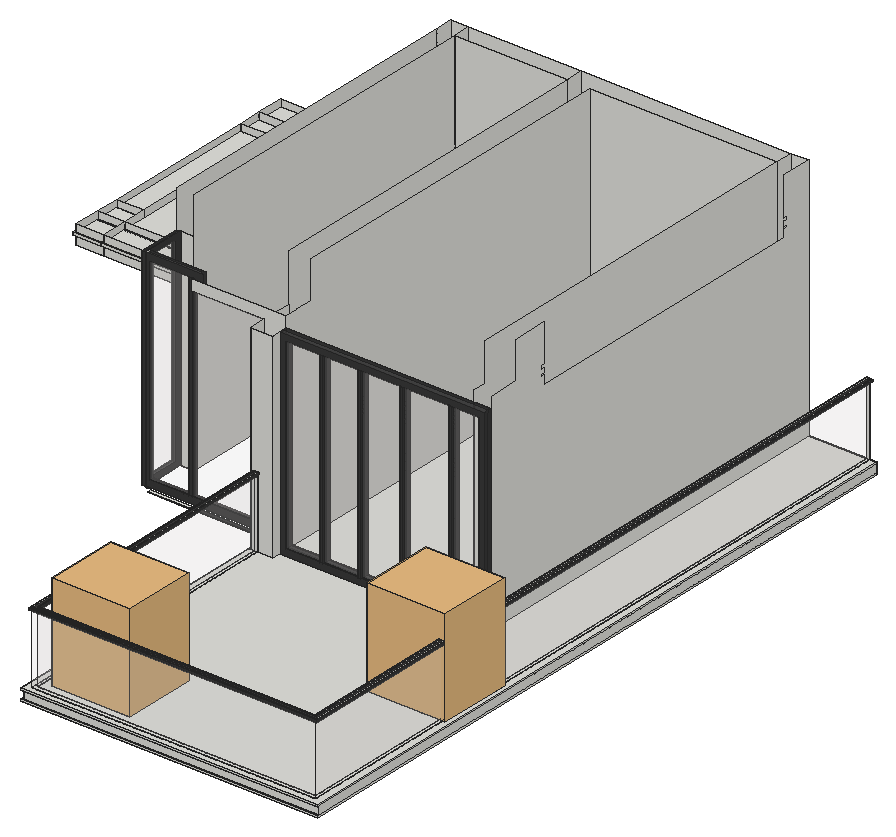
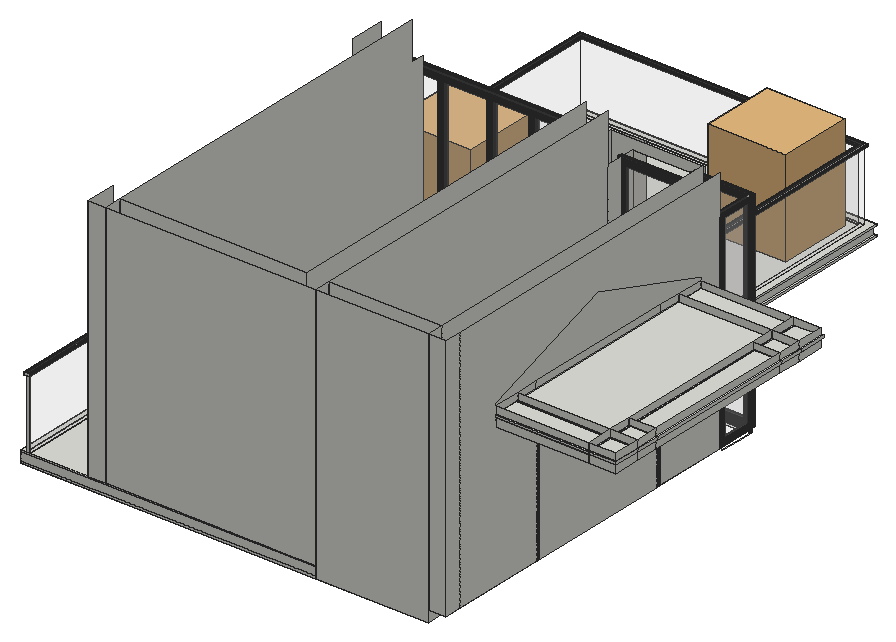
# SketchUp Ruby script. Lengths in inches.
U = 1.inch
M = Sketchup.active_model
def pt(a) = Geom::Point3d.new(a.map { |v| v * U })
def face(e, loops, mat)
  f = e.add_face(loops[0].map { |a| pt(a) })
  loops[1..].each { |l| e.add_face(l.map { |a| pt(a) }).erase! }
  f.material = f.back_material = mat if mat
  f
end
# faces: each face lists its corners as indices into pts; further lists are holes
def faces(e, pts, list, mat = nil) = list.each { |f| face(e, (f[0].is_a?(Array) ? f : [f]).map { |l| l.map { |i| pts[i] } }, mat) }
# xy, xz, yz: faces in a plane at the given z, y or x. An outline is a flat list of corners, or four numbers for a rectangle; further outlines are holes
def ring(l) = l.size == 4 ? [[l[0], l[1]], [l[2], l[1]], [l[2], l[3]], [l[0], l[3]]] : l.each_slice(2).to_a
def flat(e, list, mat, &to3) = list.each { |f| face(e, (f[0].is_a?(Array) ? f : [f]).map { |l| ring(l).map { |u, v| to3.(u, v) } }, mat) }
def xy(e, z, list, mat = nil) = flat(e, list, mat) { |x, y| [x, y, z] }
def xz(e, y, list, mat = nil) = flat(e, list, mat) { |x, z| [x, y, z] }
def yz(e, x, list, mat = nil) = flat(e, list, mat) { |y, z| [x, y, z] }
def lines(e, pts, list) = list.each { |a, b| e.add_line(pt(pts[a]), pt(pts[b])) }
# prism: a flat outline (further loops are holes) pulled along v
def prism(e, loops, v, mat = nil)
  f = face(e, loops, mat); d = Geom::Vector3d.new(v.map { |x| x * U })
  f.pushpull(f.normal.samedirection?(d) ? d.length : -d.length)
end
def box(e, o, s, mat = nil) = prism(e, [[o, [o[0] + s[0], o[1], o[2]], [o[0] + s[0], o[1] + s[1], o[2]], [o[0], o[1] + s[1], o[2]]]], [0, 0, s[2]], mat)
def at(x, y, z, deg = 0) = Geom::Transformation.translation(pt([x, y, z])) * Geom::Transformation.rotation(ORIGIN, Z_AXIS, deg.degrees)
def axes(o, x, y, z) = Geom::Transformation.new([*x, 0, *y, 0, *z, 0, *pt(o).to_a, 1])
def part(name) = M.definitions.add(name)
# library, detail: a bought-in or finely detailed component or shape, given as its bounding box
def library(name, o, s) = part(name).tap { |d| box(d.entities, o, s) }
def detail(e, o, s) = box(e.add_group.entities, o, s)
def put(e, d, t, mat = nil) = e.add_instance(d, t).tap { |i| i.material = mat if mat }
def group(e, t, mat = nil) = e.add_group.tap { |g| g.transformation = t; g.material = mat if mat }.entities
root = M.entities
M.materials.add("Glass Thin Clear 001").color = [255, 250, 250]
M.materials["Glass Thin Clear 001"].alpha = 0.1
M.materials.add("[Color M07]").color = [58, 58, 58]
c1 = library("False Aralia 002",[-20.33,-19.19,0],[40.48,38.23,49.87])
xy(root,243.5,[[208.4375,269.93,210.8125,270.37],[208.4375,270.37,210.8125,272.05]],"[Color M07]")
xy(root,246,[[208.375,108.3125,209.4375,255.6875],[209.4375,108.3125,353,109.375],[353,108.3125,362,109.375],[209.4375,109.375,353,255.6875],[353,109.375,362,469.5625],
  [208.375,255.6875,209.4375,264.6875],[209.4375,255.6875,220.8125,264.6875],[220.8125,255.6875,353,264.6875],[208.375,264.6875,209.4375,271.43],[[209.4375,264.6875,209.4375,460.5625,211.8125,460.5625,211.8125,469.5625,220.8125,469.5625,220.8125,264.6875],[210.9375,269.93,213.3125,272.05]],
  [220.8125,264.6875,353,460.5625],[208.375,271.43,209.4375,280.43],[151,460.5625,209.4375,469.5625],[209.4375,460.5625,211.8125,469.5625],[220.8125,460.5625,353,469.5625]])
xy(root,246,[[210.9375,269.93,213.3125,271.43],[210.9375,271.43,213.3125,272.05]],"[Color M07]")
xy(root,246.9375,[[208.375,108.3125,209.4375,271.43],[209.4375,108.3125,362,109.375],[209.4375,109.375,362,469.5625],[208.375,271.43,209.4375,280.43]])
xy(root,249.5,[[166.4375,269.93,168.4375,272.05],[144.9375,270.37,166.4375,272.05]])
xy(root,249.5,[[144.9375,269.93,166.4375,270.37],[168.4375,269.93,208.4375,270.37],[168.4375,270.37,208.4375,272.05]],"[Color M07]")
xy(root,250.36,[[142,272.01,142.4375,272.05],[142.4375,272.01,144.125,272.05],[142,272.05,142.4375,280.43],[142,280.43,142.4375,290.47]])
xy(root,251.125,[[208.375,108.3125,209.4375,271.43],[209.4375,108.3125,362,109.375],[209.4375,109.375,362,469.5625],[208.375,271.43,209.4375,280.43]])
xy(root,252,[[208.375,108.3125,362,108.3125,362,469.5625,358.82,469.5625,358.82,111.49,211.55,111.49,211.55,255.6875,208.375,255.6875],[211.55,111.49,211.55,255.6875,213.29,255.6875,213.29,113.23,357.09,113.23,357.09,469.5625,358.82,469.5625,358.82,111.49],[213.29,113.23,357.09,113.23,357.09,469.5625,326.84,469.5625,326.84,264.6875,220.8125,264.6875,220.8125,264.4375,326.84,264.4375,326.84,260.1875,220.8125,260.1875,220.8125,255.6875,213.29,255.6875],[208.375,255.6875,209.4375,264.6875],[209.4375,255.6875,220.8125,264.6875],
  [208.375,264.6875,209.4375,269.93],[209.4375,264.6875,209.4375,269.93,210.9375,269.93,210.9375,272.05,209.4375,272.05,209.4375,469.5625,317.84,469.5625,317.84,460.5625,220.8125,460.5625,220.8125,264.6875],[220.8125,264.6875,317.84,460.5625],[317.84,264.6875,326.84,469.5625],[209.4375,269.93,210.9375,271.43],
  [209.4375,271.43,210.9375,272.05],[208.375,272.05,209.4375,280.43],[142,292.12,151,469.5625]])
xy(root,252,[[220.8125,260.1875,317.84,262.625],[317.84,260.1875,326.84,262.625],[220.8125,262.625,317.84,264.4375],[317.84,262.625,326.84,264.4375],[142,269.93,143.5,271.43],
  [143.5,269.93,144.125,271.43],[144.125,269.93,208.375,271.43],[208.375,269.93,209.4375,271.43],[142,271.43,143.5,272.05],[143.5,271.43,144.125,272.05],
  [144.125,271.43,208.375,272.05],[208.375,271.43,209.4375,272.05],[142,272.05,143.5,280.43],[143.5,272.05,144.125,280.43],[142,280.43,143.5,292.12],
  [143.5,280.43,144.125,292.12]],"[Color M07]")
xy(root,254.83,[[142,273.2,142.4375,280.43],[142.4375,273.2,144.125,280.43],[142,280.43,142.4375,289.29],[142.4375,280.43,144.125,289.29]],"[Color M07]")
xy(root,255.11,[[241.62,260.1875,243.38,264.4375],[261.3,260.1875,263.07,264.4375],[283.05,260.1875,284.82,264.4375],[308.3125,260.1875,310.08,264.4375]])
xy(root,255.11,[[223.93,260.1875,241.62,261.1875],[243.38,260.1875,261.3,261.1875],[263.07,260.1875,283.05,261.1875],[284.82,260.1875,308.3125,261.1875],[310.08,260.1875,317.84,261.1875],
  [317.84,260.1875,323.73,261.1875],[223.93,261.1875,241.62,264.4375],[243.38,261.1875,261.3,264.4375],[263.07,261.1875,283.05,264.4375],[284.82,261.1875,308.3125,264.4375],
  [310.08,261.1875,317.84,264.4375],[317.84,261.1875,323.73,264.4375]],"[Color M07]")
xy(root,255.5,[[166.4375,269.93,168.4375,272.05]])
xy(root,255.5,[[145.94,269.93,166.4375,270.37],[168.4375,269.93,207.43,270.37],[145.94,270.37,166.4375,272.05],[168.4375,270.37,207.43,272.05]],"[Color M07]")
xy(root,288,[[211.55,111.49,211.55,255.6875,213.29,255.6875,213.29,113.23,357.09,113.23,357.09,469.5625,358.82,469.5625,358.82,111.49]])
xy(root,288,[[[210.93,110.87,210.93,256.3125,213.91,256.3125,213.91,113.85,356.46,113.85,356.46,470.1875,359.44,470.1875,359.44,110.87],[211.55,111.49,358.82,111.49,358.82,469.5625,357.09,469.5625,357.09,113.23,213.29,113.23,213.29,255.6875,211.55,255.6875]]],"[Color M07]")
xy(root,289.1875,[[[210.93,110.87,359.44,110.87,359.44,470.1875,356.46,470.1875,356.46,113.85,213.91,113.85,213.91,256.3125,210.93,256.3125],[211.55,111.49,211.55,255.6875,213.29,255.6875,213.29,113.23,357.09,113.23,357.09,469.5625,358.82,469.5625,358.82,111.49]],[211.55,111.49,358.82,111.49,358.82,469.5625,357.09,469.5625,357.09,113.23,213.29,113.23,213.29,255.6875,211.55,255.6875]],"[Color M07]")
xy(root,321.57,[[110.9,331.125,112.77,331.5625],[110.9,331.5625,112.77,332.75],[110.9,409.3125,112.77,409.75],[110.9,409.75,112.77,410.9375]])
xy(root,321.57,[[99.31,331.125,110.9,331.5625],[112.77,331.125,137.69,331.5625],[99.31,331.5625,110.9,332.75],[112.77,331.5625,137.69,332.75],[99.31,409.3125,110.9,409.75],
  [112.77,409.3125,137.69,409.75],[99.31,409.75,110.9,410.9375],[112.77,409.75,137.69,410.9375]],"[Color M07]")
xy(root,325.875,[[79.875,305,94,319.125],[94,305,142,319.125],[79.875,319.125,79.875,331.125,86,331.125,86,330.5625,94,330.5625,94,319.125],[94,319.125,94,330.5625,95,330.5625,95,331.125,142,331.125,142,319.125],[86,330.5625,94,331.125],
  [94,330.5625,95,331.125],[79.875,331.125,79.875,411.25,94,411.25,94,411.125,86,411.125,86,331.125],[86,331.125,94,411.125],[94,331.125,95,411.125],[95,332.75,142,333.43],
  [95,333.43,142,409.3125],[95,410.9375,95,411.125,94,411.125,94,411.25,142,411.25,142,410.9375],[79.875,411.25,94,423.25],[94,411.25,142,423.25],[79.875,423.25,94,437.375],
  [94,423.25,142,437.375]])
xy(root,325.875,[[95,331.125,142,332.125],[95,332.125,142,332.75],[95,409.3125,142,410.3125],[95,410.3125,142,410.9375]],"[Color M07]")
xy(root,330.53,[[79.0625,304.1875,79.0625,318.3125,79.875,318.3125,79.875,305,93.1875,305,93.1875,304.1875],[93.1875,304.1875,142,305],[79.875,305,93.1875,318.3125],[93.1875,305,94,318.3125],[94,305,142,318.3125],
  [79.0625,318.3125,79.875,319.125],[79.875,318.3125,93.1875,319.125],[93.1875,318.3125,94,319.125],[94,318.3125,142,319.125],[79.0625,319.125,79.875,331.125],
  [79.875,319.125,93.1875,331.125],[93.1875,319.125,94,331.125],[94,319.125,142,423.25],[79.0625,331.125,79.875,411.25],[79.875,331.125,93.1875,411.25],
  [93.1875,331.125,94,411.25],[79.0625,411.25,79.875,424.0625],[79.875,411.25,93.1875,423.25],[93.1875,411.25,94,423.25],[79.875,423.25,93.1875,424.0625],
  [93.1875,423.25,94,424.0625],[94,423.25,142,424.0625],[79.0625,424.0625,79.0625,438.1875,93.1875,438.1875,93.1875,437.375,79.875,437.375,79.875,424.0625],[79.875,424.0625,93.1875,437.375],[93.1875,424.0625,94,437.375],
  [94,424.0625,142,437.375],[93.1875,437.375,94,438.1875],[94,437.375,142,438.1875]])
xy(root,331.84,[[79.0625,304.1875,93.1875,304.1875,93.1875,305,79.875,305,79.875,318.3125,79.0625,318.3125],[93.1875,304.1875,142,305],[79.875,305,93.1875,318.3125],[93.1875,305,94,318.3125],[94,305,142,318.3125],
  [79.0625,318.3125,79.875,319.125],[79.875,318.3125,93.1875,319.125],[93.1875,318.3125,94,319.125],[94,318.3125,142,319.125],[79.0625,319.125,79.875,331.125],
  [79.875,319.125,93.1875,331.125],[93.1875,319.125,94,331.125],[94,319.125,142,423.25],[79.0625,331.125,79.875,411.25],[79.875,331.125,93.1875,411.25],
  [93.1875,331.125,94,411.25],[79.0625,411.25,79.875,424.0625],[79.875,411.25,93.1875,423.25],[93.1875,411.25,94,423.25],[79.875,423.25,93.1875,424.0625],
  [93.1875,423.25,94,424.0625],[94,423.25,142,424.0625],[79.0625,424.0625,79.875,424.0625,79.875,437.375,93.1875,437.375,93.1875,438.1875,79.0625,438.1875],[79.875,424.0625,93.1875,437.375],[93.1875,424.0625,94,437.375],
  [94,424.0625,142,437.375],[93.1875,437.375,94,438.1875],[94,437.375,142,438.1875]])
xz(root,108.3125,[[208.375,246,362,246.9375],[208.375,251.125,362,252]])
xz(root,109.375,[[209.4375,246.9375,362,251.125]])
xz(root,110.87,[[210.93,288,359.44,289.1875]],"[Color M07]")
xz(root,111.49,[[211.55,288,358.82,289.1875]])
xz(root,111.49,[[211.55,252,358.82,288]],"Glass Thin Clear 001")
xz(root,113.23,[[213.29,288,357.09,289.1875]])
xz(root,113.23,[[213.29,252,357.09,288]],"Glass Thin Clear 001")
xz(root,113.85,[[213.91,288,356.46,289.1875]],"[Color M07]")
xz(root,255.6875,[[209.4375,252,211.55,252,211.55,289.1875,213.29,289.1875,213.29,252,220.8125,252,220.8125,354.57,209.4375,354.57],[211.55,252,213.29,288],[211.55,288,213.29,289.1875]])
xz(root,256.3125,[[210.93,288,213.91,289.1875]])
xz(root,260.1875,[[[220.8125,252,326.84,354.57],[223.93,255.11,323.73,351.46]],[241.62,255.11,243.38,351.46],[261.3,255.11,263.07,351.46],[283.05,255.11,284.82,351.46],[308.3125,255.11,310.08,351.46]],"[Color M07]")
xz(root,261.1875,[[223.93,255.11,241.62,351.46],[243.38,255.11,261.3,351.46],[263.07,255.11,283.05,351.46],[284.82,255.11,308.3125,351.46],[310.08,255.11,323.73,351.46]],"Glass Thin Clear 001")
xz(root,262.625,[[220.8125,252,326.84,354.57]],"Glass Thin Clear 001")
xz(root,264.4375,[[[220.8125,252,326.84,354.57],[223.93,255.11,323.73,351.46]],[241.62,255.11,243.38,351.46],[261.3,255.11,263.07,351.46],[283.05,255.11,284.82,351.46],[308.3125,255.11,310.08,351.46]],"[Color M07]")
xz(root,264.6875,[[209.4375,252,209.4375,354.57,171.8125,354.57,171.8125,360,220.8125,360,220.8125,252],[317.84,252,326.84,354.57]])
xz(root,269.93,[[142,252,144.125,360.375],[[144.125,252,210.9375,252,210.9375,354.57,173.3125,354.57,173.3125,360,173.125,360,173.125,360.375,144.125,360.375],[145.94,255.5,145.94,356.87,169.62,356.87,169.62,356.5,169.81,356.5,169.81,351.07,207.43,351.07,207.43,255.5]],[166.4375,255.5,168.4375,356.87]],"[Color M07]")
xz(root,270.37,[[145.94,255.5,166.4375,356.87],[168.4375,255.5,207.43,255.5,207.43,351.07,169.81,351.07,169.81,356.5,169.62,356.5,169.62,356.87,168.4375,356.87]],"Glass Thin Clear 001")
xz(root,271.43,[[208.375,246,209.4375,246.9375],[208.375,251.125,209.4375,252]])
xz(root,271.43,[[143.5,252,143.5,360.375,171.625,360.375,171.625,360,171.8125,360,171.8125,354.57,210.9375,354.57,210.9375,252]],"Glass Thin Clear 001")
xz(root,272.05,[[142,250.36,144.125,252],[[144.125,252,144.125,360.375,173.125,360.375,173.125,360,173.3125,360,173.3125,354.57,210.9375,354.57,210.9375,252],[145.94,255.5,207.43,255.5,207.43,351.07,169.81,351.07,169.81,356.5,169.62,356.5,169.62,356.87,145.94,356.87]],[166.4375,255.5,168.4375,356.87]],"[Color M07]")
xz(root,273.2,[[142,254.83,142.4375,357.54],[142.4375,254.83,144.125,357.54]],"[Color M07]")
xz(root,280.43,[[208.375,246,209.4375,246.9375],[208.375,251.125,209.4375,252]])
xz(root,289.29,[[142,254.83,142.4375,357.54],[142.4375,254.83,144.125,357.54]],"[Color M07]")
xz(root,292.12,[[144.125,252,151,360.375]])
xz(root,292.12,[[142,252,143.5,360.375],[143.5,252,144.125,360.375]],"[Color M07]")
xz(root,304.1875,[[79.0625,330.53,93.1875,331.84],[93.1875,330.53,142,331.84]])
xz(root,305,[[79.875,325.875,94,330.53],[94,325.875,142,330.53],[79.875,331.84,94,335.4],[94,331.84,142,335.4]])
xz(root,318.3125,[[79.0625,330.53,93.1875,331.84],[93.1875,330.53,142,331.84]])
xz(root,319.125,[[79.875,325.875,94,330.53],[94,325.875,142,330.53],[79.875,331.84,94,335.4],[94,331.84,142,335.4]])
xz(root,331.125,[[79.875,325.875,94,330.53],[79.0625,330.53,93.1875,331.84],[79.875,331.84,94,335.4]])
xz(root,411.25,[[79.875,325.875,94,330.53],[79.0625,330.53,93.1875,331.84],[79.875,331.84,94,335.4]])
xz(root,423.25,[[79.875,325.875,94,330.53],[94,325.875,142,330.53],[79.875,331.84,94,335.4],[94,331.84,142,335.4]])
xz(root,424.0625,[[79.0625,330.53,93.1875,331.84],[93.1875,330.53,142,331.84]])
xz(root,437.375,[[79.875,325.875,94,330.53],[94,325.875,142,330.53],[79.875,331.84,94,335.4],[94,331.84,142,335.4]])
xz(root,438.1875,[[79.0625,330.53,93.1875,331.84],[93.1875,330.53,142,331.84]])
xz(root,460.5625,[[151,246,209.4375,379.5625],[220.8125,252,317.84,379.5625]])
xz(root,469.5625,[[151,246,209.4375,379.5625],[209.4375,246,362,246.9375],[209.4375,246.9375,362,251.125],[209.4375,251.125,362,252],[142,252,151,379.5625],
  [209.4375,252,317.84,379.5625],[317.84,252,326.84,379.5625],[357.09,252,358.82,288],[357.09,288,358.82,289.1875]])
xz(root,470.1875,[[356.46,288,359.44,289.1875]])
yz(root,79.0625,[[304.1875,330.53,318.3125,331.84],[318.3125,330.53,331.125,331.84],[331.125,330.53,411.25,331.84],[411.25,330.53,424.0625,331.84],[424.0625,330.53,438.1875,331.84]])
yz(root,79.875,[[305,325.875,319.125,330.53],[319.125,325.875,331.125,330.53],[331.125,325.875,411.25,330.53],[411.25,325.875,423.25,330.53],[423.25,325.875,437.375,330.53],
  [305,331.84,319.125,335.4],[319.125,331.84,331.125,335.4],[331.125,331.84,411.25,335.4],[411.25,331.84,423.25,335.4],[423.25,331.84,437.375,335.4]])
yz(root,93.1875,[[304.1875,330.53,318.3125,331.84],[318.3125,330.53,331.125,331.84],[331.125,330.53,411.25,331.84],[411.25,330.53,424.0625,331.84],[424.0625,330.53,438.1875,331.84]])
yz(root,94,[[305,325.875,319.125,330.53],[319.125,325.875,331.125,330.53],[331.125,325.875,411.25,330.53],[411.25,325.875,423.25,330.53],[423.25,325.875,437.375,330.53],
  [305,331.84,319.125,335.4],[319.125,331.84,331.125,335.4],[331.125,331.84,411.25,335.4],[411.25,331.84,423.25,335.4],[423.25,331.84,437.375,335.4]])
yz(root,142,[[292.12,252,292.12,379.5625,460.5625,379.5625,460.5625,252,410.9375,252,410.9375,325.875,437.375,325.875,437.375,330.53,438.1875,330.53,438.1875,331.84,437.375,331.84,437.375,335.4,438.1875,335.4,438.1875,336.97,371.1875,359.28,304.1875,336.97,304.1875,335.4,305,335.4,305,331.84,304.1875,331.84,304.1875,330.53,305,330.53,305,325.875,331.125,325.875,331.125,252],[332.75,252,333.43,325.875],[333.43,252,409.3125,325.875],[460.5625,252,469.5625,379.5625],[305,325.875,319.125,330.53],
  [319.125,325.875,331.125,330.53],[331.125,325.875,411.25,330.53],[411.25,325.875,423.25,330.53],[423.25,325.875,437.375,330.53],[304.1875,330.53,318.3125,331.84],
  [318.3125,330.53,331.125,331.84],[331.125,330.53,411.25,331.84],[411.25,330.53,424.0625,331.84],[424.0625,330.53,438.1875,331.84],[305,331.84,319.125,335.4],
  [319.125,331.84,331.125,335.4],[331.125,331.84,411.25,335.4],[411.25,331.84,423.25,335.4],[423.25,331.84,437.375,335.4]])
yz(root,142,[[[269.93,252,292.12,360.375],[273.2,254.83,289.29,357.54]],[331.125,252,332.125,325.875],[332.125,252,332.75,325.875],[409.3125,252,410.3125,325.875],[410.3125,252,410.9375,325.875]],"[Color M07]")
yz(root,142.4375,[[273.2,254.83,289.29,357.54]],"Glass Thin Clear 001")
yz(root,143.5,[[270.37,252,271.43,360.375],[271.43,252,292.12,360.375]],"Glass Thin Clear 001")
yz(root,144.125,[[269.93,252,272.05,360.375]])
yz(root,144.125,[[[272.05,252,292.12,360.375],[273.2,254.83,289.29,357.54]]],"[Color M07]")
yz(root,145.94,[[269.93,255.5,270.37,356.87],[270.37,255.5,272.05,356.87]],"[Color M07]")
yz(root,151,[[460.5625,246,469.5625,252],[292.12,252,460.5625,379.5625],[460.5625,252,469.5625,379.5625]])
yz(root,166.4375,[[269.93,255.5,270.37,356.87],[270.37,255.5,272.05,356.87]],"[Color M07]")
yz(root,168.4375,[[269.93,255.5,270.37,356.87],[270.37,255.5,272.05,356.87]],"[Color M07]")
yz(root,207.43,[[269.93,255.5,270.37,351.07],[270.37,255.5,272.05,351.07]],"[Color M07]")
yz(root,208.375,[[108.3125,246,271.43,246.9375],[271.43,246,280.43,246.9375],[108.3125,251.125,271.43,252],[271.43,251.125,280.43,252]])
yz(root,208.4375,[[269.93,243.5,270.37,246.9375],[270.37,243.5,272.05,246.9375],[269.93,246.9375,270.37,249.5],[270.37,246.9375,272.05,249.5]],"[Color M07]")
yz(root,209.4375,[[271.43,246,280.43,246.9375],[280.43,246,460.5625,246.9375],[460.5625,246,469.5625,246.9375],[109.375,246.9375,280.43,251.125],[280.43,246.9375,460.5625,251.125],
  [460.5625,246.9375,469.5625,251.125],[271.43,251.125,280.43,252],[280.43,251.125,460.5625,252],[460.5625,251.125,469.5625,252],[255.6875,252,264.6875,354.57],
  [264.6875,252,280.43,354.57],[280.43,252,460.5625,379.5625],[460.5625,252,469.5625,379.5625]])
yz(root,210.93,[[110.87,288,256.3125,289.1875]],"[Color M07]")
yz(root,210.9375,[[269.93,246,271.43,246.9375],[271.43,246,272.05,246.9375],[269.93,246.9375,271.43,251.125],[271.43,246.9375,272.05,251.125],[269.93,251.125,271.43,252],
  [271.43,251.125,272.05,252],[269.93,252,271.43,354.57],[271.43,252,272.05,354.57]],"[Color M07]")
yz(root,211.55,[[111.49,288,255.6875,289.1875]])
yz(root,211.55,[[111.49,252,255.6875,288]],"Glass Thin Clear 001")
yz(root,213.29,[[113.23,288,255.6875,289.1875]])
yz(root,213.29,[[113.23,252,255.6875,288]],"Glass Thin Clear 001")
yz(root,213.91,[[113.85,288,256.3125,289.1875]],"[Color M07]")
yz(root,220.8125,[[255.6875,252,260.1875,354.57],[264.4375,252,264.6875,354.57],[264.6875,252,460.5625,252,460.5625,379.5625,280.43,379.5625,280.43,360.375,271.43,360.375,271.43,360,264.6875,360]])
yz(root,220.8125,[[260.1875,252,262.625,354.57],[262.625,252,264.4375,354.57]],"[Color M07]")
yz(root,223.93,[[260.1875,255.11,261.1875,351.46],[261.1875,255.11,264.4375,351.46]],"[Color M07]")
yz(root,241.62,[[260.1875,255.11,261.1875,351.46],[261.1875,255.11,264.4375,351.46]],"[Color M07]")
yz(root,243.38,[[260.1875,255.11,261.1875,351.46],[261.1875,255.11,264.4375,351.46]],"[Color M07]")
yz(root,261.3,[[260.1875,255.11,261.1875,351.46],[261.1875,255.11,264.4375,351.46]],"[Color M07]")
yz(root,263.07,[[260.1875,255.11,261.1875,351.46],[261.1875,255.11,264.4375,351.46]],"[Color M07]")
yz(root,283.05,[[260.1875,255.11,261.1875,351.46],[261.1875,255.11,264.4375,351.46]],"[Color M07]")
yz(root,284.82,[[260.1875,255.11,261.1875,351.46],[261.1875,255.11,264.4375,351.46]],"[Color M07]")
yz(root,308.3125,[[260.1875,255.11,261.1875,351.46],[261.1875,255.11,264.4375,351.46]],"[Color M07]")
yz(root,310.08,[[260.1875,255.11,261.1875,351.46],[261.1875,255.11,264.4375,351.46]],"[Color M07]")
yz(root,317.84,[[264.6875,252,264.6875,360,271.43,360,271.43,379.5625,460.5625,379.5625,460.5625,252],[460.5625,252,469.5625,379.5625]])
yz(root,323.73,[[260.1875,255.11,261.1875,351.46],[261.1875,255.11,264.4375,351.46]],"[Color M07]")
yz(root,326.84,[[264.6875,252,469.5625,252,469.5625,379.5625,453.63,379.5625,453.63,360,455.51,360,455.51,358.3125,453.63,358.3125,453.63,355.8125,455.51,355.8125,455.51,354.9375,453.63,354.9375,453.63,350.5625,298.82,350.5625,298.82,354.9375,296.95,354.9375,296.95,355.8125,298.82,355.8125,298.82,358.3125,296.95,358.3125,296.95,360,298.82,360,298.82,379.5625,280.43,379.5625,280.43,360.375,271.43,360.375,271.43,360,264.6875,360]])
yz(root,326.84,[[260.1875,252,262.625,354.57],[262.625,252,264.4375,354.57]],"[Color M07]")
yz(root,356.46,[[113.85,288,470.1875,289.1875]],"[Color M07]")
yz(root,357.09,[[113.23,288,469.5625,289.1875]])
yz(root,357.09,[[113.23,252,469.5625,288]],"Glass Thin Clear 001")
yz(root,358.82,[[111.49,288,469.5625,289.1875]])
yz(root,358.82,[[111.49,252,469.5625,288]],"Glass Thin Clear 001")
yz(root,359.44,[[110.87,288,470.1875,289.1875]],"[Color M07]")
yz(root,362,[[108.3125,246,469.5625,246.9375],[109.375,246.9375,469.5625,251.125],[108.3125,251.125,469.5625,252]])
p = [[209.4375,280.43,246],[211.8125,280.43,246]]
lines(root,p,[[0,1]])
put(root,c1,at(237.34,136.82,252))
put(root,c1,at(339.41,213.1875,252))
